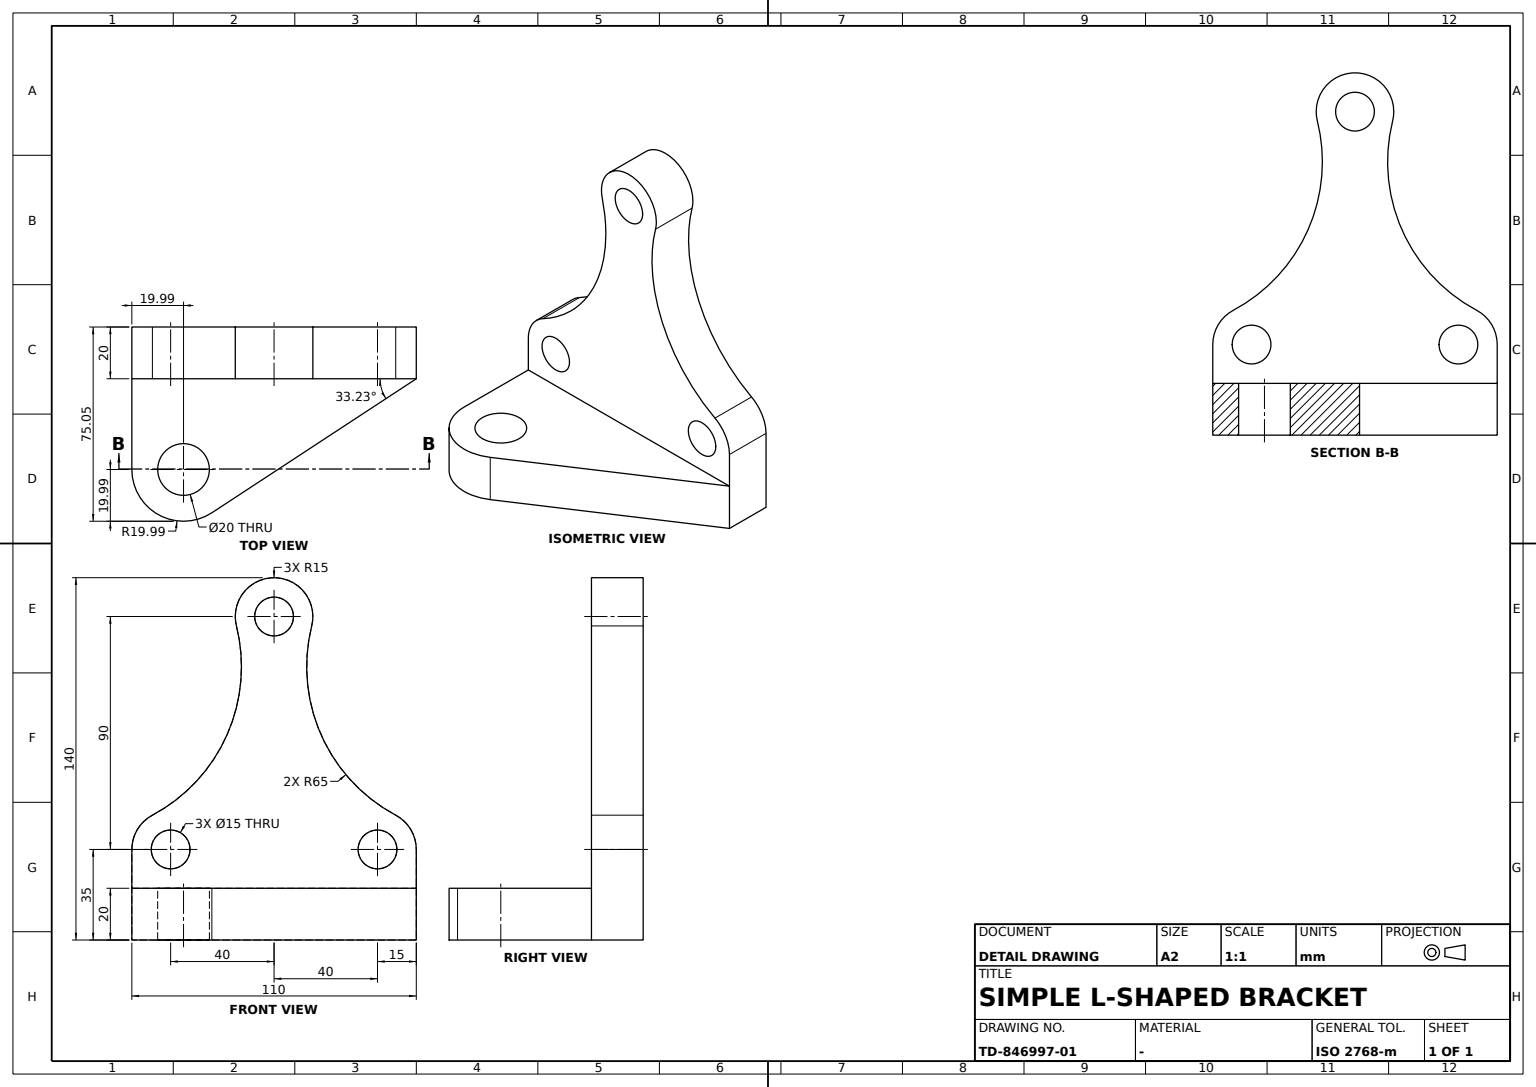
ISO-10303-21;
HEADER;
FILE_DESCRIPTION((''),'2;1');
FILE_NAME('','',(''),(''),'','','');
FILE_SCHEMA(('AUTOMOTIVE_DESIGN'));
ENDSEC;
DATA;
#1=APPLICATION_CONTEXT('');
#2=PRODUCT_CONTEXT('',#1,'mechanical');
#3=PRODUCT('','','',(#2));
#4=PRODUCT_DEFINITION_FORMATION('','',#3);
#5=PRODUCT_DEFINITION_CONTEXT('',#1,'design');
#6=PRODUCT_DEFINITION('','',#4,#5);
#7=PRODUCT_DEFINITION_SHAPE('','',#6);
#8=(LENGTH_UNIT()NAMED_UNIT(*)SI_UNIT(.MILLI.,.METRE.));
#9=(NAMED_UNIT(*)PLANE_ANGLE_UNIT()SI_UNIT($,.RADIAN.));
#10=(NAMED_UNIT(*)SI_UNIT($,.STERADIAN.)SOLID_ANGLE_UNIT());
#11=UNCERTAINTY_MEASURE_WITH_UNIT(LENGTH_MEASURE(1.E-05),#8,'distance_accuracy_value','');
#12=(GEOMETRIC_REPRESENTATION_CONTEXT(3)GLOBAL_UNCERTAINTY_ASSIGNED_CONTEXT((#11))GLOBAL_UNIT_ASSIGNED_CONTEXT((#8,#9,#10))REPRESENTATION_CONTEXT('',''));
#13=CARTESIAN_POINT('',(0.,-32.5,0.));
#14=VERTEX_POINT('',#13);
#15=CARTESIAN_POINT('',(20.,-32.5,0.));
#16=VERTEX_POINT('',#15);
#17=CARTESIAN_POINT('',(10.,-32.5,0.));
#18=DIRECTION('',(1.,0.,0.));
#19=VECTOR('',#18,1000.);
#20=LINE('',#17,#19);
#21=EDGE_CURVE('',#14,#16,#20,.T.);
#22=ORIENTED_EDGE('',*,*,#21,.T.);
#23=CARTESIAN_POINT('',(20.,-47.5,0.));
#24=VERTEX_POINT('',#23);
#25=CARTESIAN_POINT('',(20.,-40.,0.));
#26=DIRECTION('',(0.,1.,0.));
#27=AXIS2_PLACEMENT_3D('',#25,#18,#26);
#28=CIRCLE('',#27,7.5);
#29=EDGE_CURVE('',#16,#24,#28,.T.);
#30=ORIENTED_EDGE('',*,*,#29,.T.);
#31=CARTESIAN_POINT('',(0.,-47.5,0.));
#32=VERTEX_POINT('',#31);
#33=CARTESIAN_POINT('',(10.,-47.5,0.));
#34=LINE('',#33,#19);
#35=EDGE_CURVE('',#32,#24,#34,.T.);
#36=ORIENTED_EDGE('',*,*,#35,.F.);
#37=CARTESIAN_POINT('',(0.,-40.,0.));
#38=AXIS2_PLACEMENT_3D('',#37,#18,#26);
#39=CIRCLE('',#38,7.5);
#40=EDGE_CURVE('',#14,#32,#39,.T.);
#41=ORIENTED_EDGE('',*,*,#40,.F.);
#42=EDGE_LOOP('',(#22,#30,#36,#41));
#43=FACE_OUTER_BOUND('',#42,.T.);
#44=CARTESIAN_POINT('',(10.,-40.,0.));
#45=DIRECTION('',(-1.,0.,0.));
#46=AXIS2_PLACEMENT_3D('',#44,#45,#26);
#47=CYLINDRICAL_SURFACE('',#46,7.5);
#48=ADVANCED_FACE('',(#43),#47,.F.);
#49=CARTESIAN_POINT('',(0.,55.,0.));
#50=VERTEX_POINT('',#49);
#51=CARTESIAN_POINT('',(20.,55.,0.));
#52=VERTEX_POINT('',#51);
#53=CARTESIAN_POINT('',(10.,55.,0.));
#54=LINE('',#53,#19);
#55=EDGE_CURVE('',#50,#52,#54,.T.);
#56=ORIENTED_EDGE('',*,*,#55,.T.);
#57=CARTESIAN_POINT('',(20.,55.,-15.));
#58=VERTEX_POINT('',#57);
#59=CARTESIAN_POINT('',(20.,55.,-7.5));
#60=DIRECTION('',(0.,0.,1.));
#61=VECTOR('',#60,1000.);
#62=LINE('',#59,#61);
#63=EDGE_CURVE('',#58,#52,#62,.T.);
#64=ORIENTED_EDGE('',*,*,#63,.F.);
#65=CARTESIAN_POINT('',(20.,55.,-35.));
#66=VERTEX_POINT('',#65);
#67=CARTESIAN_POINT('',(20.,55.,-25.));
#68=LINE('',#67,#61);
#69=EDGE_CURVE('',#66,#58,#68,.T.);
#70=ORIENTED_EDGE('',*,*,#69,.F.);
#71=CARTESIAN_POINT('',(0.,55.,-35.));
#72=VERTEX_POINT('',#71);
#73=CARTESIAN_POINT('',(10.,55.,-35.));
#74=LINE('',#73,#19);
#75=EDGE_CURVE('',#72,#66,#74,.T.);
#76=ORIENTED_EDGE('',*,*,#75,.F.);
#77=CARTESIAN_POINT('',(0.,55.,-17.5));
#78=LINE('',#77,#61);
#79=EDGE_CURVE('',#72,#50,#78,.T.);
#80=ORIENTED_EDGE('',*,*,#79,.T.);
#81=EDGE_LOOP('',(#56,#64,#70,#76,#80));
#82=FACE_OUTER_BOUND('',#81,.T.);
#83=DIRECTION('',(0.,-1.,0.));
#84=DIRECTION('',(0.,0.,-1.));
#85=AXIS2_PLACEMENT_3D('',#49,#83,#84);
#86=PLANE('',#85);
#87=ADVANCED_FACE('',(#82),#86,.F.);
#88=CARTESIAN_POINT('',(0.,-14.552555,86.363635));
#89=VERTEX_POINT('',#88);
#90=CARTESIAN_POINT('',(20.,-14.552555,86.363635));
#91=VERTEX_POINT('',#90);
#92=CARTESIAN_POINT('',(10.,-14.552555,86.363635));
#93=LINE('',#92,#19);
#94=EDGE_CURVE('',#89,#91,#93,.T.);
#95=ORIENTED_EDGE('',*,*,#94,.F.);
#96=CARTESIAN_POINT('',(0.,-12.613626,70.606056));
#97=VERTEX_POINT('',#96);
#98=CARTESIAN_POINT('',(0.,-77.613626,70.606056));
#99=AXIS2_PLACEMENT_3D('',#98,#45,#26);
#100=CIRCLE('',#99,65.);
#101=EDGE_CURVE('',#89,#97,#100,.T.);
#102=ORIENTED_EDGE('',*,*,#101,.T.);
#103=CARTESIAN_POINT('',(20.,-12.613626,70.606056));
#104=VERTEX_POINT('',#103);
#105=CARTESIAN_POINT('',(10.,-12.613626,70.606056));
#106=VECTOR('',#45,1000.);
#107=LINE('',#105,#106);
#108=EDGE_CURVE('',#104,#97,#107,.T.);
#109=ORIENTED_EDGE('',*,*,#108,.F.);
#110=CARTESIAN_POINT('',(20.,-77.613626,70.606056));
#111=AXIS2_PLACEMENT_3D('',#110,#45,#26);
#112=CIRCLE('',#111,65.);
#113=EDGE_CURVE('',#91,#104,#112,.T.);
#114=ORIENTED_EDGE('',*,*,#113,.F.);
#115=EDGE_LOOP('',(#95,#102,#109,#114));
#116=FACE_OUTER_BOUND('',#115,.T.);
#117=CARTESIAN_POINT('',(10.,-77.613626,70.606056));
#118=AXIS2_PLACEMENT_3D('',#117,#45,#26);
#119=CYLINDRICAL_SURFACE('',#118,65.);
#120=ADVANCED_FACE('',(#116),#119,.F.);
#121=ORIENTED_EDGE('',*,*,#35,.T.);
#122=EDGE_CURVE('',#24,#16,#28,.T.);
#123=ORIENTED_EDGE('',*,*,#122,.T.);
#124=ORIENTED_EDGE('',*,*,#21,.F.);
#125=EDGE_CURVE('',#32,#14,#39,.T.);
#126=ORIENTED_EDGE('',*,*,#125,.F.);
#127=EDGE_LOOP('',(#121,#123,#124,#126));
#128=FACE_OUTER_BOUND('',#127,.T.);
#129=ADVANCED_FACE('',(#128),#47,.F.);
#130=CARTESIAN_POINT('',(0.,-47.052555,13.238635));
#131=VERTEX_POINT('',#130);
#132=CARTESIAN_POINT('',(20.,-47.052555,13.238635));
#133=VERTEX_POINT('',#132);
#134=CARTESIAN_POINT('',(10.,-47.052555,13.238635));
#135=LINE('',#134,#19);
#136=EDGE_CURVE('',#131,#133,#135,.T.);
#137=ORIENTED_EDGE('',*,*,#136,.F.);
#138=CARTESIAN_POINT('',(0.,-55.,0.));
#139=VERTEX_POINT('',#138);
#140=CIRCLE('',#38,15.);
#141=EDGE_CURVE('',#131,#139,#140,.T.);
#142=ORIENTED_EDGE('',*,*,#141,.T.);
#143=CARTESIAN_POINT('',(20.,-55.,0.));
#144=VERTEX_POINT('',#143);
#145=CARTESIAN_POINT('',(10.,-55.,0.));
#146=LINE('',#145,#19);
#147=EDGE_CURVE('',#139,#144,#146,.T.);
#148=ORIENTED_EDGE('',*,*,#147,.T.);
#149=CIRCLE('',#27,15.);
#150=EDGE_CURVE('',#133,#144,#149,.T.);
#151=ORIENTED_EDGE('',*,*,#150,.F.);
#152=EDGE_LOOP('',(#137,#142,#148,#151));
#153=FACE_OUTER_BOUND('',#152,.T.);
#154=CYLINDRICAL_SURFACE('',#46,15.);
#155=ADVANCED_FACE('',(#153),#154,.T.);
#156=CARTESIAN_POINT('',(71.784022,-24.054571,-35.));
#157=VERTEX_POINT('',#156);
#158=CARTESIAN_POINT('',(45.892011,15.472715,-35.));
#159=DIRECTION('',(0.547949614,-0.836511339,0.));
#160=VECTOR('',#159,1000.);
#161=LINE('',#158,#160);
#162=EDGE_CURVE('',#66,#157,#161,.T.);
#163=ORIENTED_EDGE('',*,*,#162,.F.);
#164=ORIENTED_EDGE('',*,*,#69,.T.);
#165=CARTESIAN_POINT('',(71.784022,-24.054571,-15.));
#166=VERTEX_POINT('',#165);
#167=CARTESIAN_POINT('',(45.892011,15.472715,-15.));
#168=LINE('',#167,#160);
#169=EDGE_CURVE('',#58,#166,#168,.T.);
#170=ORIENTED_EDGE('',*,*,#169,.T.);
#171=CARTESIAN_POINT('',(71.784022,-24.054571,-25.));
#172=LINE('',#171,#61);
#173=EDGE_CURVE('',#157,#166,#172,.T.);
#174=ORIENTED_EDGE('',*,*,#173,.F.);
#175=EDGE_LOOP('',(#163,#164,#170,#174));
#176=FACE_OUTER_BOUND('',#175,.T.);
#177=DIRECTION('',(-0.836511339,-0.547949614,0.));
#178=AXIS2_PLACEMENT_3D('',#65,#177,#159);
#179=PLANE('',#178);
#180=ADVANCED_FACE('',(#176),#179,.F.);
#181=CARTESIAN_POINT('',(20.,32.5,0.));
#182=VERTEX_POINT('',#181);
#183=CARTESIAN_POINT('',(20.,47.5,0.));
#184=VERTEX_POINT('',#183);
#185=CARTESIAN_POINT('',(20.,40.,0.));
#186=AXIS2_PLACEMENT_3D('',#185,#18,#26);
#187=CIRCLE('',#186,7.5);
#188=EDGE_CURVE('',#182,#184,#187,.T.);
#189=ORIENTED_EDGE('',*,*,#188,.T.);
#190=CARTESIAN_POINT('',(0.,47.5,0.));
#191=VERTEX_POINT('',#190);
#192=CARTESIAN_POINT('',(10.,47.5,0.));
#193=LINE('',#192,#19);
#194=EDGE_CURVE('',#191,#184,#193,.T.);
#195=ORIENTED_EDGE('',*,*,#194,.F.);
#196=CARTESIAN_POINT('',(0.,32.5,0.));
#197=VERTEX_POINT('',#196);
#198=CARTESIAN_POINT('',(0.,40.,0.));
#199=AXIS2_PLACEMENT_3D('',#198,#18,#26);
#200=CIRCLE('',#199,7.5);
#201=EDGE_CURVE('',#197,#191,#200,.T.);
#202=ORIENTED_EDGE('',*,*,#201,.F.);
#203=CARTESIAN_POINT('',(10.,32.5,0.));
#204=LINE('',#203,#19);
#205=EDGE_CURVE('',#197,#182,#204,.T.);
#206=ORIENTED_EDGE('',*,*,#205,.T.);
#207=EDGE_LOOP('',(#189,#195,#202,#206));
#208=FACE_OUTER_BOUND('',#207,.T.);
#209=CARTESIAN_POINT('',(10.,40.,0.));
#210=AXIS2_PLACEMENT_3D('',#209,#45,#26);
#211=CYLINDRICAL_SURFACE('',#210,7.5);
#212=ADVANCED_FACE('',(#208),#211,.F.);
#213=CARTESIAN_POINT('',(45.061125,-35.008762,-15.));
#214=VERTEX_POINT('',#213);
#215=CARTESIAN_POINT('',(65.061125,-35.008762,-15.));
#216=VERTEX_POINT('',#215);
#217=CARTESIAN_POINT('',(55.061125,-35.008762,-15.));
#218=AXIS2_PLACEMENT_3D('',#217,#84,#18);
#219=CIRCLE('',#218,10.);
#220=EDGE_CURVE('',#214,#216,#219,.T.);
#221=ORIENTED_EDGE('',*,*,#220,.F.);
#222=CARTESIAN_POINT('',(45.061125,-35.008762,-35.));
#223=VERTEX_POINT('',#222);
#224=CARTESIAN_POINT('',(45.061125,-35.008762,-25.));
#225=LINE('',#224,#61);
#226=EDGE_CURVE('',#223,#214,#225,.T.);
#227=ORIENTED_EDGE('',*,*,#226,.F.);
#228=CARTESIAN_POINT('',(65.061125,-35.008762,-35.));
#229=VERTEX_POINT('',#228);
#230=CARTESIAN_POINT('',(55.061125,-35.008762,-35.));
#231=AXIS2_PLACEMENT_3D('',#230,#84,#18);
#232=CIRCLE('',#231,10.);
#233=EDGE_CURVE('',#223,#229,#232,.T.);
#234=ORIENTED_EDGE('',*,*,#233,.T.);
#235=CARTESIAN_POINT('',(65.061125,-35.008762,-25.));
#236=LINE('',#235,#61);
#237=EDGE_CURVE('',#229,#216,#236,.T.);
#238=ORIENTED_EDGE('',*,*,#237,.T.);
#239=EDGE_LOOP('',(#221,#227,#234,#238));
#240=FACE_OUTER_BOUND('',#239,.T.);
#241=CARTESIAN_POINT('',(55.061125,-35.008762,-25.));
#242=AXIS2_PLACEMENT_3D('',#241,#60,#18);
#243=CYLINDRICAL_SURFACE('',#242,10.);
#244=ADVANCED_FACE('',(#240),#243,.F.);
#245=ORIENTED_EDGE('',*,*,#75,.T.);
#246=ORIENTED_EDGE('',*,*,#162,.T.);
#247=CARTESIAN_POINT('',(75.052363,-35.008762,-35.));
#248=VERTEX_POINT('',#247);
#249=CIRCLE('',#231,19.991238);
#250=EDGE_CURVE('',#157,#248,#249,.T.);
#251=ORIENTED_EDGE('',*,*,#250,.T.);
#252=CARTESIAN_POINT('',(55.061125,-55.,-35.));
#253=VERTEX_POINT('',#252);
#254=EDGE_CURVE('',#248,#253,#249,.T.);
#255=ORIENTED_EDGE('',*,*,#254,.T.);
#256=CARTESIAN_POINT('',(0.,-55.,-35.));
#257=VERTEX_POINT('',#256);
#258=CARTESIAN_POINT('',(27.530562,-55.,-35.));
#259=LINE('',#258,#19);
#260=EDGE_CURVE('',#257,#253,#259,.T.);
#261=ORIENTED_EDGE('',*,*,#260,.F.);
#262=CARTESIAN_POINT('',(0.,0.,-35.));
#263=VECTOR('',#26,1000.);
#264=LINE('',#262,#263);
#265=EDGE_CURVE('',#257,#72,#264,.T.);
#266=ORIENTED_EDGE('',*,*,#265,.T.);
#267=EDGE_LOOP('',(#245,#246,#251,#255,#261,#266));
#268=FACE_OUTER_BOUND('',#267,.T.);
#269=EDGE_CURVE('',#229,#223,#232,.T.);
#270=ORIENTED_EDGE('',*,*,#269,.F.);
#271=ORIENTED_EDGE('',*,*,#233,.F.);
#272=EDGE_LOOP('',(#270,#271));
#273=FACE_BOUND('',#272,.T.);
#274=AXIS2_PLACEMENT_3D('',#256,#84,#26);
#275=PLANE('',#274);
#276=ADVANCED_FACE('',(#268,#273),#275,.T.);
#277=ORIENTED_EDGE('',*,*,#29,.F.);
#278=ORIENTED_EDGE('',*,*,#122,.F.);
#279=EDGE_LOOP('',(#277,#278));
#280=FACE_BOUND('',#279,.T.);
#281=CARTESIAN_POINT('',(20.,-55.,-15.));
#282=VERTEX_POINT('',#281);
#283=CARTESIAN_POINT('',(20.,0.,-15.));
#284=LINE('',#283,#263);
#285=EDGE_CURVE('',#282,#58,#284,.T.);
#286=ORIENTED_EDGE('',*,*,#285,.T.);
#287=ORIENTED_EDGE('',*,*,#63,.T.);
#288=CARTESIAN_POINT('',(20.,47.052555,13.238635));
#289=VERTEX_POINT('',#288);
#290=CIRCLE('',#186,15.);
#291=EDGE_CURVE('',#52,#289,#290,.T.);
#292=ORIENTED_EDGE('',*,*,#291,.T.);
#293=CARTESIAN_POINT('',(20.,14.552555,86.363635));
#294=VERTEX_POINT('',#293);
#295=CARTESIAN_POINT('',(20.,77.613626,70.606056));
#296=AXIS2_PLACEMENT_3D('',#295,#45,#26);
#297=CIRCLE('',#296,65.);
#298=EDGE_CURVE('',#289,#294,#297,.T.);
#299=ORIENTED_EDGE('',*,*,#298,.T.);
#300=CARTESIAN_POINT('',(20.,15.,90.));
#301=VERTEX_POINT('',#300);
#302=CARTESIAN_POINT('',(20.,0.,90.));
#303=AXIS2_PLACEMENT_3D('',#302,#18,#26);
#304=CIRCLE('',#303,15.);
#305=EDGE_CURVE('',#294,#301,#304,.T.);
#306=ORIENTED_EDGE('',*,*,#305,.T.);
#307=CARTESIAN_POINT('',(20.,-15.,90.));
#308=VERTEX_POINT('',#307);
#309=EDGE_CURVE('',#301,#308,#304,.T.);
#310=ORIENTED_EDGE('',*,*,#309,.T.);
#311=EDGE_CURVE('',#308,#91,#304,.T.);
#312=ORIENTED_EDGE('',*,*,#311,.T.);
#313=ORIENTED_EDGE('',*,*,#113,.T.);
#314=EDGE_CURVE('',#104,#133,#112,.T.);
#315=ORIENTED_EDGE('',*,*,#314,.T.);
#316=ORIENTED_EDGE('',*,*,#150,.T.);
#317=CARTESIAN_POINT('',(20.,-55.,-7.5));
#318=VECTOR('',#84,1000.);
#319=LINE('',#317,#318);
#320=EDGE_CURVE('',#144,#282,#319,.T.);
#321=ORIENTED_EDGE('',*,*,#320,.T.);
#322=EDGE_LOOP('',(#286,#287,#292,#299,#306,#310,#312,#313,#315,#316,#321));
#323=FACE_OUTER_BOUND('',#322,.T.);
#324=ORIENTED_EDGE('',*,*,#188,.F.);
#325=EDGE_CURVE('',#184,#182,#187,.T.);
#326=ORIENTED_EDGE('',*,*,#325,.F.);
#327=EDGE_LOOP('',(#324,#326));
#328=FACE_BOUND('',#327,.T.);
#329=CARTESIAN_POINT('',(20.,7.5,90.));
#330=VERTEX_POINT('',#329);
#331=CARTESIAN_POINT('',(20.,-7.5,90.));
#332=VERTEX_POINT('',#331);
#333=CIRCLE('',#303,7.5);
#334=EDGE_CURVE('',#330,#332,#333,.T.);
#335=ORIENTED_EDGE('',*,*,#334,.F.);
#336=EDGE_CURVE('',#332,#330,#333,.T.);
#337=ORIENTED_EDGE('',*,*,#336,.F.);
#338=EDGE_LOOP('',(#335,#337));
#339=FACE_BOUND('',#338,.T.);
#340=CARTESIAN_POINT('',(20.,0.,0.));
#341=AXIS2_PLACEMENT_3D('',#340,#18,#26);
#342=PLANE('',#341);
#343=ADVANCED_FACE('',(#280,#323,#328,#339),#342,.T.);
#344=ORIENTED_EDGE('',*,*,#325,.T.);
#345=ORIENTED_EDGE('',*,*,#205,.F.);
#346=EDGE_CURVE('',#191,#197,#200,.T.);
#347=ORIENTED_EDGE('',*,*,#346,.F.);
#348=ORIENTED_EDGE('',*,*,#194,.T.);
#349=EDGE_LOOP('',(#344,#345,#347,#348));
#350=FACE_OUTER_BOUND('',#349,.T.);
#351=ADVANCED_FACE('',(#350),#211,.F.);
#352=ORIENTED_EDGE('',*,*,#40,.T.);
#353=ORIENTED_EDGE('',*,*,#125,.T.);
#354=EDGE_LOOP('',(#352,#353));
#355=FACE_BOUND('',#354,.T.);
#356=CARTESIAN_POINT('',(0.,-15.,90.));
#357=VERTEX_POINT('',#356);
#358=CARTESIAN_POINT('',(0.,0.,90.));
#359=AXIS2_PLACEMENT_3D('',#358,#18,#26);
#360=CIRCLE('',#359,15.);
#361=EDGE_CURVE('',#357,#89,#360,.T.);
#362=ORIENTED_EDGE('',*,*,#361,.F.);
#363=CARTESIAN_POINT('',(0.,15.,90.));
#364=VERTEX_POINT('',#363);
#365=EDGE_CURVE('',#364,#357,#360,.T.);
#366=ORIENTED_EDGE('',*,*,#365,.F.);
#367=CARTESIAN_POINT('',(0.,14.552555,86.363635));
#368=VERTEX_POINT('',#367);
#369=EDGE_CURVE('',#368,#364,#360,.T.);
#370=ORIENTED_EDGE('',*,*,#369,.F.);
#371=CARTESIAN_POINT('',(0.,47.052555,13.238635));
#372=VERTEX_POINT('',#371);
#373=CARTESIAN_POINT('',(0.,77.613626,70.606056));
#374=AXIS2_PLACEMENT_3D('',#373,#45,#26);
#375=CIRCLE('',#374,65.);
#376=EDGE_CURVE('',#372,#368,#375,.T.);
#377=ORIENTED_EDGE('',*,*,#376,.F.);
#378=CIRCLE('',#199,15.);
#379=EDGE_CURVE('',#50,#372,#378,.T.);
#380=ORIENTED_EDGE('',*,*,#379,.F.);
#381=ORIENTED_EDGE('',*,*,#79,.F.);
#382=ORIENTED_EDGE('',*,*,#265,.F.);
#383=CARTESIAN_POINT('',(0.,-55.,-17.5));
#384=LINE('',#383,#318);
#385=EDGE_CURVE('',#139,#257,#384,.T.);
#386=ORIENTED_EDGE('',*,*,#385,.F.);
#387=ORIENTED_EDGE('',*,*,#141,.F.);
#388=EDGE_CURVE('',#97,#131,#100,.T.);
#389=ORIENTED_EDGE('',*,*,#388,.F.);
#390=ORIENTED_EDGE('',*,*,#101,.F.);
#391=EDGE_LOOP('',(#362,#366,#370,#377,#380,#381,#382,#386,#387,#389,#390));
#392=FACE_OUTER_BOUND('',#391,.T.);
#393=CARTESIAN_POINT('',(0.,-7.5,90.));
#394=VERTEX_POINT('',#393);
#395=CARTESIAN_POINT('',(0.,7.5,90.));
#396=VERTEX_POINT('',#395);
#397=CIRCLE('',#359,7.5);
#398=EDGE_CURVE('',#394,#396,#397,.T.);
#399=ORIENTED_EDGE('',*,*,#398,.T.);
#400=EDGE_CURVE('',#396,#394,#397,.T.);
#401=ORIENTED_EDGE('',*,*,#400,.T.);
#402=EDGE_LOOP('',(#399,#401));
#403=FACE_BOUND('',#402,.T.);
#404=ORIENTED_EDGE('',*,*,#346,.T.);
#405=ORIENTED_EDGE('',*,*,#201,.T.);
#406=EDGE_LOOP('',(#404,#405));
#407=FACE_BOUND('',#406,.T.);
#408=CARTESIAN_POINT('',(0.,0.,0.));
#409=AXIS2_PLACEMENT_3D('',#408,#18,#26);
#410=PLANE('',#409);
#411=ADVANCED_FACE('',(#355,#392,#403,#407),#410,.F.);
#412=CARTESIAN_POINT('',(75.052363,-35.008762,-15.));
#413=VERTEX_POINT('',#412);
#414=CARTESIAN_POINT('',(75.052363,-35.008762,-25.));
#415=LINE('',#414,#61);
#416=EDGE_CURVE('',#248,#413,#415,.T.);
#417=ORIENTED_EDGE('',*,*,#416,.T.);
#418=CARTESIAN_POINT('',(55.061125,-55.,-15.));
#419=VERTEX_POINT('',#418);
#420=CIRCLE('',#218,19.991238);
#421=EDGE_CURVE('',#413,#419,#420,.T.);
#422=ORIENTED_EDGE('',*,*,#421,.T.);
#423=CARTESIAN_POINT('',(55.061125,-55.,-25.));
#424=LINE('',#423,#61);
#425=EDGE_CURVE('',#253,#419,#424,.T.);
#426=ORIENTED_EDGE('',*,*,#425,.F.);
#427=ORIENTED_EDGE('',*,*,#254,.F.);
#428=EDGE_LOOP('',(#417,#422,#426,#427));
#429=FACE_OUTER_BOUND('',#428,.T.);
#430=CYLINDRICAL_SURFACE('',#242,19.991238);
#431=ADVANCED_FACE('',(#429),#430,.T.);
#432=ORIENTED_EDGE('',*,*,#173,.T.);
#433=EDGE_CURVE('',#166,#413,#420,.T.);
#434=ORIENTED_EDGE('',*,*,#433,.T.);
#435=ORIENTED_EDGE('',*,*,#416,.F.);
#436=ORIENTED_EDGE('',*,*,#250,.F.);
#437=EDGE_LOOP('',(#432,#434,#435,#436));
#438=FACE_OUTER_BOUND('',#437,.T.);
#439=ADVANCED_FACE('',(#438),#430,.T.);
#440=ORIENTED_EDGE('',*,*,#311,.F.);
#441=CARTESIAN_POINT('',(10.,-15.,90.));
#442=LINE('',#441,#106);
#443=EDGE_CURVE('',#308,#357,#442,.T.);
#444=ORIENTED_EDGE('',*,*,#443,.T.);
#445=ORIENTED_EDGE('',*,*,#361,.T.);
#446=ORIENTED_EDGE('',*,*,#94,.T.);
#447=EDGE_LOOP('',(#440,#444,#445,#446));
#448=FACE_OUTER_BOUND('',#447,.T.);
#449=CARTESIAN_POINT('',(10.,0.,90.));
#450=AXIS2_PLACEMENT_3D('',#449,#45,#26);
#451=CYLINDRICAL_SURFACE('',#450,15.);
#452=ADVANCED_FACE('',(#448),#451,.T.);
#453=ORIENTED_EDGE('',*,*,#400,.F.);
#454=CARTESIAN_POINT('',(10.,7.5,90.));
#455=LINE('',#454,#19);
#456=EDGE_CURVE('',#396,#330,#455,.T.);
#457=ORIENTED_EDGE('',*,*,#456,.T.);
#458=ORIENTED_EDGE('',*,*,#334,.T.);
#459=CARTESIAN_POINT('',(10.,-7.5,90.));
#460=LINE('',#459,#19);
#461=EDGE_CURVE('',#394,#332,#460,.T.);
#462=ORIENTED_EDGE('',*,*,#461,.F.);
#463=EDGE_LOOP('',(#453,#457,#458,#462));
#464=FACE_OUTER_BOUND('',#463,.T.);
#465=CYLINDRICAL_SURFACE('',#450,7.5);
#466=ADVANCED_FACE('',(#464),#465,.F.);
#467=ORIENTED_EDGE('',*,*,#388,.T.);
#468=ORIENTED_EDGE('',*,*,#136,.T.);
#469=ORIENTED_EDGE('',*,*,#314,.F.);
#470=ORIENTED_EDGE('',*,*,#108,.T.);
#471=EDGE_LOOP('',(#467,#468,#469,#470));
#472=FACE_OUTER_BOUND('',#471,.T.);
#473=ADVANCED_FACE('',(#472),#119,.F.);
#474=ORIENTED_EDGE('',*,*,#309,.F.);
#475=CARTESIAN_POINT('',(10.,15.,90.));
#476=LINE('',#475,#106);
#477=EDGE_CURVE('',#301,#364,#476,.T.);
#478=ORIENTED_EDGE('',*,*,#477,.T.);
#479=ORIENTED_EDGE('',*,*,#365,.T.);
#480=ORIENTED_EDGE('',*,*,#443,.F.);
#481=EDGE_LOOP('',(#474,#478,#479,#480));
#482=FACE_OUTER_BOUND('',#481,.T.);
#483=ADVANCED_FACE('',(#482),#451,.T.);
#484=CARTESIAN_POINT('',(10.,47.052555,13.238635));
#485=LINE('',#484,#19);
#486=EDGE_CURVE('',#372,#289,#485,.T.);
#487=ORIENTED_EDGE('',*,*,#486,.T.);
#488=ORIENTED_EDGE('',*,*,#291,.F.);
#489=ORIENTED_EDGE('',*,*,#55,.F.);
#490=ORIENTED_EDGE('',*,*,#379,.T.);
#491=EDGE_LOOP('',(#487,#488,#489,#490));
#492=FACE_OUTER_BOUND('',#491,.T.);
#493=CYLINDRICAL_SURFACE('',#210,15.);
#494=ADVANCED_FACE('',(#492),#493,.T.);
#495=ORIENTED_EDGE('',*,*,#237,.F.);
#496=ORIENTED_EDGE('',*,*,#269,.T.);
#497=ORIENTED_EDGE('',*,*,#226,.T.);
#498=EDGE_CURVE('',#216,#214,#219,.T.);
#499=ORIENTED_EDGE('',*,*,#498,.F.);
#500=EDGE_LOOP('',(#495,#496,#497,#499));
#501=FACE_OUTER_BOUND('',#500,.T.);
#502=ADVANCED_FACE('',(#501),#243,.F.);
#503=ORIENTED_EDGE('',*,*,#433,.F.);
#504=ORIENTED_EDGE('',*,*,#169,.F.);
#505=ORIENTED_EDGE('',*,*,#285,.F.);
#506=CARTESIAN_POINT('',(37.530562,-55.,-15.));
#507=LINE('',#506,#106);
#508=EDGE_CURVE('',#419,#282,#507,.T.);
#509=ORIENTED_EDGE('',*,*,#508,.F.);
#510=ORIENTED_EDGE('',*,*,#421,.F.);
#511=EDGE_LOOP('',(#503,#504,#505,#509,#510));
#512=FACE_OUTER_BOUND('',#511,.T.);
#513=ORIENTED_EDGE('',*,*,#220,.T.);
#514=ORIENTED_EDGE('',*,*,#498,.T.);
#515=EDGE_LOOP('',(#513,#514));
#516=FACE_BOUND('',#515,.T.);
#517=CARTESIAN_POINT('',(0.,0.,-15.));
#518=AXIS2_PLACEMENT_3D('',#517,#84,#18);
#519=PLANE('',#518);
#520=ADVANCED_FACE('',(#512,#516),#519,.F.);
#521=ORIENTED_EDGE('',*,*,#320,.F.);
#522=ORIENTED_EDGE('',*,*,#147,.F.);
#523=ORIENTED_EDGE('',*,*,#385,.T.);
#524=ORIENTED_EDGE('',*,*,#260,.T.);
#525=ORIENTED_EDGE('',*,*,#425,.T.);
#526=ORIENTED_EDGE('',*,*,#508,.T.);
#527=EDGE_LOOP('',(#521,#522,#523,#524,#525,#526));
#528=FACE_OUTER_BOUND('',#527,.T.);
#529=AXIS2_PLACEMENT_3D('',#138,#83,#84);
#530=PLANE('',#529);
#531=ADVANCED_FACE('',(#528),#530,.T.);
#532=ORIENTED_EDGE('',*,*,#336,.T.);
#533=ORIENTED_EDGE('',*,*,#456,.F.);
#534=ORIENTED_EDGE('',*,*,#398,.F.);
#535=ORIENTED_EDGE('',*,*,#461,.T.);
#536=EDGE_LOOP('',(#532,#533,#534,#535));
#537=FACE_OUTER_BOUND('',#536,.T.);
#538=ADVANCED_FACE('',(#537),#465,.F.);
#539=ORIENTED_EDGE('',*,*,#477,.F.);
#540=ORIENTED_EDGE('',*,*,#305,.F.);
#541=CARTESIAN_POINT('',(10.,14.552555,86.363635));
#542=LINE('',#541,#19);
#543=EDGE_CURVE('',#368,#294,#542,.T.);
#544=ORIENTED_EDGE('',*,*,#543,.F.);
#545=ORIENTED_EDGE('',*,*,#369,.T.);
#546=EDGE_LOOP('',(#539,#540,#544,#545));
#547=FACE_OUTER_BOUND('',#546,.T.);
#548=ADVANCED_FACE('',(#547),#451,.T.);
#549=ORIENTED_EDGE('',*,*,#543,.T.);
#550=ORIENTED_EDGE('',*,*,#298,.F.);
#551=ORIENTED_EDGE('',*,*,#486,.F.);
#552=ORIENTED_EDGE('',*,*,#376,.T.);
#553=EDGE_LOOP('',(#549,#550,#551,#552));
#554=FACE_OUTER_BOUND('',#553,.T.);
#555=CARTESIAN_POINT('',(10.,77.613626,70.606056));
#556=AXIS2_PLACEMENT_3D('',#555,#45,#26);
#557=CYLINDRICAL_SURFACE('',#556,65.);
#558=ADVANCED_FACE('',(#554),#557,.F.);
#559=CLOSED_SHELL('',(#48,#87,#120,#129,#155,#180,#212,#244,#276,#343,#351,#411,#431,#439,#452,#466,#473,#483,#494,#502,#520,#531,#538,#548,#558));
#560=MANIFOLD_SOLID_BREP('',#559);
#561=ADVANCED_BREP_SHAPE_REPRESENTATION('',(#560),#12);
#562=SHAPE_DEFINITION_REPRESENTATION(#7,#561);
ENDSEC;
END-ISO-10303-21;
